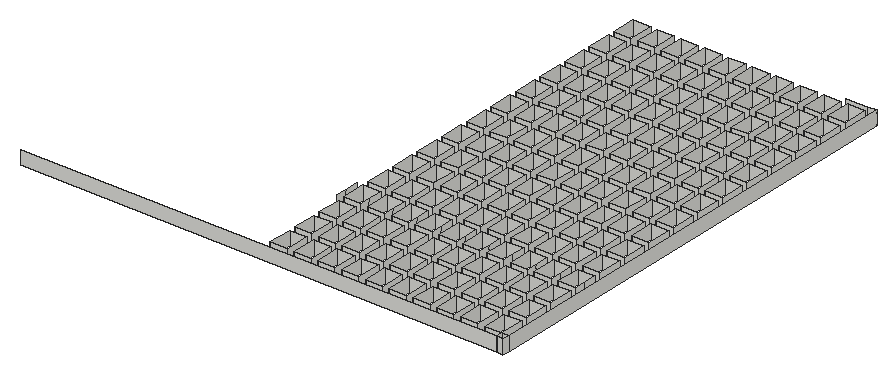
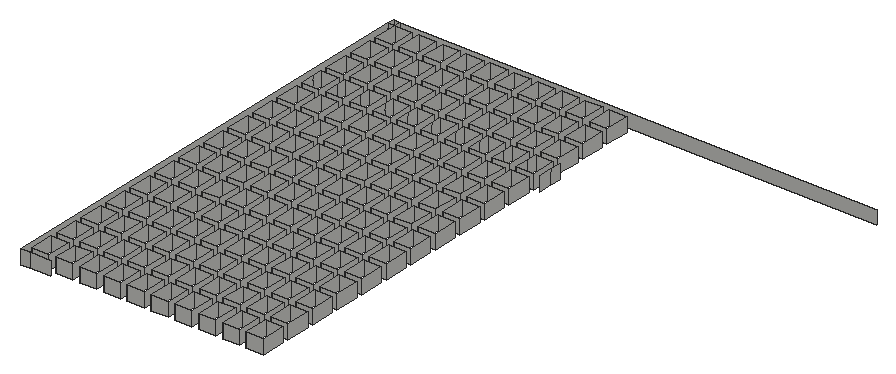
# SketchUp Ruby script. Lengths in inches.
U = 1.inch
M = Sketchup.active_model
def pt(a) = Geom::Point3d.new(a.map { |v| v * U })
def face(e, loops, mat)
  f = e.add_face(loops[0].map { |a| pt(a) })
  loops[1..].each { |l| e.add_face(l.map { |a| pt(a) }).erase! }
  f.material = f.back_material = mat if mat
  f
end
# faces: each face lists its corners as indices into pts; further lists are holes
def faces(e, pts, list, mat = nil) = list.each { |f| face(e, (f[0].is_a?(Array) ? f : [f]).map { |l| l.map { |i| pts[i] } }, mat) }
# xy, xz, yz: faces in a plane at the given z, y or x. An outline is a flat list of corners, or four numbers for a rectangle; further outlines are holes
def ring(l) = l.size == 4 ? [[l[0], l[1]], [l[2], l[1]], [l[2], l[3]], [l[0], l[3]]] : l.each_slice(2).to_a
def flat(e, list, mat, &to3) = list.each { |f| face(e, (f[0].is_a?(Array) ? f : [f]).map { |l| ring(l).map { |u, v| to3.(u, v) } }, mat) }
def xy(e, z, list, mat = nil) = flat(e, list, mat) { |x, y| [x, y, z] }
def xz(e, y, list, mat = nil) = flat(e, list, mat) { |x, z| [x, y, z] }
def yz(e, x, list, mat = nil) = flat(e, list, mat) { |y, z| [x, y, z] }
def lines(e, pts, list) = list.each { |a, b| e.add_line(pt(pts[a]), pt(pts[b])) }
# prism: a flat outline (further loops are holes) pulled along v
def prism(e, loops, v, mat = nil)
  f = face(e, loops, mat); d = Geom::Vector3d.new(v.map { |x| x * U })
  f.pushpull(f.normal.samedirection?(d) ? d.length : -d.length)
end
def box(e, o, s, mat = nil) = prism(e, [[o, [o[0] + s[0], o[1], o[2]], [o[0] + s[0], o[1] + s[1], o[2]], [o[0], o[1] + s[1], o[2]]]], [0, 0, s[2]], mat)
def at(x, y, z, deg = 0) = Geom::Transformation.translation(pt([x, y, z])) * Geom::Transformation.rotation(ORIGIN, Z_AXIS, deg.degrees)
def axes(o, x, y, z) = Geom::Transformation.new([*x, 0, *y, 0, *z, 0, *pt(o).to_a, 1])
def part(name) = M.definitions.add(name)
# library, detail: a bought-in or finely detailed component or shape, given as its bounding box
def library(name, o, s) = part(name).tap { |d| box(d.entities, o, s) }
def detail(e, o, s) = box(e.add_group.entities, o, s)
def put(e, d, t, mat = nil) = e.add_instance(d, t).tap { |i| i.material = mat if mat }
def group(e, t, mat = nil) = e.add_group.tap { |g| g.transformation = t; g.material = mat if mat }.entities
root = M.entities
xy(root,246,[[589.58,38.27,589.58,51.29,582.19,51.29,582.19,41,592.3,41,592.3,38.27]])
xz(root,38.27,[[387.37,246,589.58,252],[589.58,246,592.3,252]])
xz(root,41,[[491.2,246,498.58,252],[501.31,246,508.69,252],[511.42,246,518.8,252],[521.53,246,528.91,252],[531.64,246,539.02,252],
  [541.75,246,549.13,252],[551.86,246,559.24,252],[561.97,246,569.35,252],[572.08,246,579.47,252],[582.19,246,589.58,252],
  [589.58,246,592.3,252]])
xz(root,51.29,[[491.2,246,498.58,252],[501.31,246,508.69,252],[511.42,246,518.8,252],[521.53,246,528.91,252],[531.64,246,539.02,252],
  [541.75,246,549.13,252],[551.86,246,559.24,252],[561.97,246,569.35,252],[572.08,246,579.47,252],[582.19,246,589.58,252]])
xz(root,54.01,[[491.2,246,498.58,252],[501.31,246,508.69,252],[511.42,246,518.8,252],[521.53,246,528.91,252],[531.64,246,539.02,252],
  [541.75,246,549.13,252],[551.86,246,559.24,252],[561.97,246,569.35,252],[572.08,246,579.47,252],[582.19,246,589.58,252]])
xz(root,64.3,[[491.2,246,498.58,252],[501.31,246,508.69,252],[511.42,246,518.8,252],[521.53,246,528.91,252],[531.64,246,539.02,252],
  [541.75,246,549.13,252],[551.86,246,559.24,252],[561.97,246,569.35,252],[572.08,246,579.47,252],[582.19,246,589.58,252]])
xz(root,67.02,[[491.2,246,498.58,252],[501.31,246,508.69,252],[511.42,246,518.8,252],[521.53,246,528.91,252],[531.64,246,539.02,252],
  [541.75,246,549.13,252],[551.86,246,559.24,252],[561.97,246,569.35,252],[572.08,246,579.47,252],[582.19,246,589.58,252]])
xz(root,77.31,[[491.2,246,498.58,252],[501.31,246,508.69,252],[511.42,246,518.8,252],[521.53,246,528.91,252],[531.64,246,539.02,252],
  [541.75,246,549.13,252],[551.86,246,559.24,252],[561.97,246,569.35,252],[572.08,246,579.47,252],[582.19,246,589.58,252]])
xz(root,80.03,[[491.2,246,498.58,252],[501.31,246,508.69,252],[511.42,246,518.8,252],[521.53,246,528.91,252],[531.64,246,539.02,252],
  [541.75,246,549.13,252],[551.86,246,559.24,252],[561.97,246,569.35,252],[572.08,246,579.47,252],[582.19,246,589.58,252]])
xz(root,90.32,[[491.2,246,498.58,252],[501.31,246,508.69,252],[511.42,246,518.8,252],[521.53,246,528.91,252],[531.64,246,539.02,252],
  [541.75,246,549.13,252],[551.86,246,559.24,252],[561.97,246,569.35,252],[572.08,246,579.47,252],[582.19,246,589.58,252]])
xz(root,93.05,[[491.2,246,498.58,252],[501.31,246,508.69,252],[511.42,246,518.8,252],[521.53,246,528.91,252],[531.64,246,539.02,252],
  [541.75,246,549.13,252],[551.86,246,559.24,252],[561.97,246,569.35,252],[572.08,246,579.47,252],[582.19,246,589.58,252]])
xz(root,103.33,[[491.2,246,498.58,252],[501.31,246,508.69,252],[511.42,246,518.8,252],[521.53,246,528.91,252],[531.64,246,539.02,252],
  [541.75,246,549.13,252],[551.86,246,559.24,252],[561.97,246,569.35,252],[572.08,246,579.47,252],[582.19,246,589.58,252]])
xz(root,106.06,[[491.2,246,498.58,252],[501.31,246,508.69,252],[511.42,246,518.8,252],[521.53,246,528.91,252],[531.64,246,539.02,252],
  [541.75,246,549.13,252],[551.86,246,559.24,252],[561.97,246,569.35,252],[572.08,246,579.47,252],[582.19,246,589.58,252]])
xz(root,116.34,[[491.2,246,498.58,252],[501.31,246,508.69,252],[511.42,246,518.8,252],[521.53,246,528.91,252],[531.64,246,539.02,252],
  [541.75,246,549.13,252],[551.86,246,559.24,252],[561.97,246,569.35,252],[572.08,246,579.47,252],[582.19,246,589.58,252]])
xz(root,119.07,[[491.2,246,498.58,252],[501.31,246,508.69,252],[511.42,246,518.8,252],[521.53,246,528.91,252],[531.64,246,539.02,252],
  [541.75,246,549.13,252],[551.86,246,559.24,252],[561.97,246,569.35,252],[572.08,246,579.47,252],[582.19,246,589.58,252]])
xz(root,129.36,[[491.2,246,498.58,252],[501.31,246,508.69,252],[511.42,246,518.8,252],[521.53,246,528.91,252],[531.64,246,539.02,252],
  [541.75,246,549.13,252],[551.86,246,559.24,252],[561.97,246,569.35,252],[572.08,246,579.47,252],[582.19,246,589.58,252]])
xz(root,132.08,[[491.2,246,498.58,252],[501.31,246,508.69,252],[511.42,246,518.8,252],[521.53,246,528.91,252],[531.64,246,539.02,252],
  [541.75,246,549.13,252],[551.86,246,559.24,252],[561.97,246,569.35,252],[572.08,246,579.47,252],[582.19,246,589.58,252]])
xz(root,142.37,[[491.2,246,498.58,252],[501.31,246,508.69,252],[511.42,246,518.8,252],[521.53,246,528.91,252],[531.64,246,539.02,252],
  [541.75,246,549.13,252],[551.86,246,559.24,252],[561.97,246,569.35,252],[572.08,246,579.47,252],[582.19,246,589.58,252]])
xz(root,145.09,[[491.2,246,498.58,252],[501.31,246,508.69,252],[511.42,246,518.8,252],[521.53,246,528.91,252],[531.64,246,539.02,252],
  [541.75,246,549.13,252],[551.86,246,559.24,252],[561.97,246,569.35,252],[572.08,246,579.47,252],[582.19,246,589.58,252]])
xz(root,155.38,[[491.2,246,498.58,252],[501.31,246,508.69,252],[511.42,246,518.8,252],[521.53,246,528.91,252],[531.64,246,539.02,252],
  [541.75,246,549.13,252],[551.86,246,559.24,252],[561.97,246,569.35,252],[572.08,246,579.47,252],[582.19,246,589.58,252]])
xz(root,158.1,[[491.2,246,498.58,252],[501.31,246,508.69,252],[511.42,246,518.8,252],[521.53,246,528.91,252],[531.64,246,539.02,252],
  [541.75,246,549.13,252],[551.86,246,559.24,252],[561.97,246,569.35,252],[572.08,246,579.47,252],[582.19,246,589.58,252]])
xz(root,168.39,[[491.2,246,498.58,252],[501.31,246,508.69,252],[511.42,246,518.8,252],[521.53,246,528.91,252],[531.64,246,539.02,252],
  [541.75,246,549.13,252],[551.86,246,559.24,252],[561.97,246,569.35,252],[572.08,246,579.47,252],[582.19,246,589.58,252]])
xz(root,171.12,[[491.2,246,498.58,252],[501.31,246,508.69,252],[511.42,246,518.8,252],[521.53,246,528.91,252],[531.64,246,539.02,252],
  [541.75,246,549.13,252],[551.86,246,559.24,252],[561.97,246,569.35,252],[572.08,246,579.47,252],[582.19,246,589.58,252]])
xz(root,181.4,[[491.2,246,498.58,252],[501.31,246,508.69,252],[511.42,246,518.8,252],[521.53,246,528.91,252],[531.64,246,539.02,252],
  [541.75,246,549.13,252],[551.86,246,559.24,252],[561.97,246,569.35,252],[572.08,246,579.47,252],[582.19,246,589.58,252]])
xz(root,184.13,[[491.2,246,498.58,252],[501.31,246,508.69,252],[511.42,246,518.8,252],[521.53,246,528.91,252],[531.64,246,539.02,252],
  [541.75,246,549.13,252],[551.86,246,559.24,252],[561.97,246,569.35,252],[572.08,246,579.47,252],[582.19,246,589.58,252]])
xz(root,194.41,[[491.2,246,498.58,252],[501.31,246,508.69,252],[511.42,246,518.8,252],[521.53,246,528.91,252],[531.64,246,539.02,252],
  [541.75,246,549.13,252],[551.86,246,559.24,252],[561.97,246,569.35,252],[572.08,246,579.47,252],[582.19,246,589.58,252]])
xz(root,197.14,[[491.2,246,498.58,252],[501.31,246,508.69,252],[511.42,246,518.8,252],[521.53,246,528.91,252],[531.64,246,539.02,252],
  [541.75,246,549.13,252],[551.86,246,559.24,252],[561.97,246,569.35,252],[572.08,246,579.47,252],[582.19,246,589.58,252]])
xz(root,207.43,[[491.2,246,498.58,252],[501.31,246,508.69,252],[511.42,246,518.8,252],[521.53,246,528.91,252],[531.64,246,539.02,252],
  [541.75,246,549.13,252],[551.86,246,559.24,252],[561.97,246,569.35,252],[572.08,246,579.47,252],[582.19,246,589.58,252]])
xz(root,210.15,[[491.2,246,498.58,252],[501.31,246,508.69,252],[511.42,246,518.8,252],[521.53,246,528.91,252],[531.64,246,539.02,252],
  [541.75,246,549.13,252],[551.86,246,559.24,252],[561.97,246,569.35,252],[572.08,246,579.47,252],[582.19,246,589.58,252]])
xz(root,220.4375,[[491.2,246,498.58,252],[501.31,246,508.69,252],[511.42,246,518.8,252],[521.53,246,528.91,252],[531.64,246,539.02,252],
  [541.75,246,549.13,252],[551.86,246,559.24,252],[561.97,246,569.35,252],[572.08,246,579.47,252],[582.19,246,589.58,252]])
xz(root,223.16,[[491.2,246,498.58,252],[501.31,246,508.69,252],[511.42,246,518.8,252],[521.53,246,528.91,252],[531.64,246,539.02,252],
  [541.75,246,549.13,252],[551.86,246,559.24,252],[561.97,246,569.35,252],[572.08,246,579.47,252],[582.19,246,589.58,252]])
xz(root,233.45,[[491.2,246,498.58,252],[501.31,246,508.69,252],[511.42,246,518.8,252],[521.53,246,528.91,252],[531.64,246,539.02,252],
  [541.75,246,549.13,252],[551.86,246,559.24,252],[561.97,246,569.35,252],[572.08,246,579.47,252],[582.19,246,589.58,252]])
xz(root,236.18,[[579.37,246,588.37,252],[588.37,246,592.3,252]])
yz(root,488.47,[[80.03,246,84.36,252],[84.36,246,90.32,252]])
yz(root,491.2,[[41,246,51.29,252],[54.01,246,64.3,252],[67.02,246,77.31,252],[80.03,246,90.32,252],[93.05,246,103.33,252],
  [106.06,246,116.34,252],[119.07,246,129.36,252],[132.08,246,142.37,252],[145.09,246,155.38,252],[158.1,246,168.39,252],
  [171.12,246,181.4,252],[184.13,246,194.41,252],[197.14,246,207.43,252],[210.15,246,220.4375,252],[223.16,246,233.45,252]])
yz(root,498.58,[[41,246,51.29,252],[54.01,246,64.3,252],[67.02,246,77.31,252],[80.03,246,84.36,252],[84.36,246,90.32,252],
  [93.05,246,103.33,252],[106.06,246,116.34,252],[119.07,246,129.36,252],[132.08,246,142.37,252],[145.09,246,155.38,252],
  [158.1,246,168.39,252],[171.12,246,181.4,252],[184.13,246,194.41,252],[197.14,246,207.43,252],[210.15,246,220.4375,252],
  [223.16,246,233.45,252]])
yz(root,501.31,[[41,246,51.29,252],[54.01,246,64.3,252],[67.02,246,77.31,252],[80.03,246,90.32,252],[93.05,246,103.33,252],
  [106.06,246,116.34,252],[119.07,246,129.36,252],[132.08,246,142.37,252],[145.09,246,155.38,252],[158.1,246,168.39,252],
  [171.12,246,181.4,252],[184.13,246,194.41,252],[197.14,246,207.43,252],[210.15,246,220.4375,252],[223.16,246,233.45,252]])
yz(root,508.69,[[41,246,51.29,252],[54.01,246,64.3,252],[67.02,246,77.31,252],[80.03,246,84.36,252],[84.36,246,90.32,252],
  [93.05,246,103.33,252],[106.06,246,116.34,252],[119.07,246,129.36,252],[132.08,246,142.37,252],[145.09,246,155.38,252],
  [158.1,246,168.39,252],[171.12,246,181.4,252],[184.13,246,194.41,252],[197.14,246,207.43,252],[210.15,246,220.4375,252],
  [223.16,246,233.45,252]])
yz(root,511.42,[[41,246,51.29,252],[54.01,246,64.3,252],[67.02,246,77.31,252],[80.03,246,90.32,252],[93.05,246,103.33,252],
  [106.06,246,116.34,252],[119.07,246,129.36,252],[132.08,246,142.37,252],[145.09,246,155.38,252],[158.1,246,168.39,252],
  [171.12,246,181.4,252],[184.13,246,194.41,252],[197.14,246,207.43,252],[210.15,246,220.4375,252],[223.16,246,233.45,252]])
yz(root,518.8,[[41,246,51.29,252],[54.01,246,64.3,252],[67.02,246,77.31,252],[80.03,246,84.36,252],[84.36,246,90.32,252],
  [93.05,246,103.33,252],[106.06,246,116.34,252],[119.07,246,129.36,252],[132.08,246,142.37,252],[145.09,246,155.38,252],
  [158.1,246,168.39,252],[171.12,246,181.4,252],[184.13,246,194.41,252],[197.14,246,207.43,252],[210.15,246,220.4375,252],
  [223.16,246,233.45,252]])
yz(root,521.53,[[41,246,51.29,252],[54.01,246,64.3,252],[67.02,246,77.31,252],[80.03,246,90.32,252],[93.05,246,103.33,252],
  [106.06,246,116.34,252],[119.07,246,129.36,252],[132.08,246,142.37,252],[145.09,246,155.38,252],[158.1,246,168.39,252],
  [171.12,246,181.4,252],[184.13,246,194.41,252],[197.14,246,207.43,252],[210.15,246,220.4375,252],[223.16,246,233.45,252]])
yz(root,528.91,[[41,246,51.29,252],[54.01,246,64.3,252],[67.02,246,77.31,252],[80.03,246,84.36,252],[84.36,246,90.32,252],
  [93.05,246,103.33,252],[106.06,246,116.34,252],[119.07,246,129.36,252],[132.08,246,142.37,252],[145.09,246,155.38,252],
  [158.1,246,168.39,252],[171.12,246,181.4,252],[184.13,246,194.41,252],[197.14,246,207.43,252],[210.15,246,220.4375,252],
  [223.16,246,233.45,252]])
yz(root,531.64,[[41,246,51.29,252],[54.01,246,64.3,252],[67.02,246,77.31,252],[80.03,246,90.32,252],[93.05,246,103.33,252],
  [106.06,246,116.34,252],[119.07,246,129.36,252],[132.08,246,142.37,252],[145.09,246,155.38,252],[158.1,246,168.39,252],
  [171.12,246,181.4,252],[184.13,246,194.41,252],[197.14,246,207.43,252],[210.15,246,220.4375,252],[223.16,246,233.45,252]])
yz(root,539.02,[[41,246,51.29,252],[54.01,246,64.3,252],[67.02,246,77.31,252],[80.03,246,84.36,252],[84.36,246,90.32,252],
  [93.05,246,103.33,252],[106.06,246,116.34,252],[119.07,246,129.36,252],[132.08,246,142.37,252],[145.09,246,155.38,252],
  [158.1,246,168.39,252],[171.12,246,181.4,252],[184.13,246,194.41,252],[197.14,246,207.43,252],[210.15,246,220.4375,252],
  [223.16,246,233.45,252]])
yz(root,541.75,[[41,246,51.29,252],[54.01,246,64.3,252],[67.02,246,77.31,252],[80.03,246,90.32,252],[93.05,246,103.33,252],
  [106.06,246,116.34,252],[119.07,246,129.36,252],[132.08,246,142.37,252],[145.09,246,155.38,252],[158.1,246,168.39,252],
  [171.12,246,181.4,252],[184.13,246,194.41,252],[197.14,246,207.43,252],[210.15,246,220.4375,252],[223.16,246,233.45,252]])
yz(root,549.13,[[41,246,51.29,252],[54.01,246,64.3,252],[67.02,246,77.31,252],[80.03,246,84.36,252],[84.36,246,90.32,252],
  [93.05,246,103.33,252],[106.06,246,116.34,252],[119.07,246,129.36,252],[132.08,246,142.37,252],[145.09,246,155.38,252],
  [158.1,246,168.39,252],[171.12,246,181.4,252],[184.13,246,194.41,252],[197.14,246,207.43,252],[210.15,246,220.4375,252],
  [223.16,246,233.45,252]])
yz(root,551.86,[[41,246,51.29,252],[54.01,246,64.3,252],[67.02,246,77.31,252],[80.03,246,90.32,252],[93.05,246,103.33,252],
  [106.06,246,116.34,252],[119.07,246,129.36,252],[132.08,246,142.37,252],[145.09,246,155.38,252],[158.1,246,168.39,252],
  [171.12,246,181.4,252],[184.13,246,194.41,252],[197.14,246,207.43,252],[210.15,246,220.4375,252],[223.16,246,233.45,252]])
yz(root,559.24,[[41,246,51.29,252],[54.01,246,64.3,252],[67.02,246,77.31,252],[80.03,246,84.36,252],[84.36,246,90.32,252],
  [93.05,246,103.33,252],[106.06,246,116.34,252],[119.07,246,129.36,252],[132.08,246,142.37,252],[145.09,246,155.38,252],
  [158.1,246,168.39,252],[171.12,246,181.4,252],[184.13,246,194.41,252],[197.14,246,207.43,252],[210.15,246,220.4375,252],
  [223.16,246,233.45,252]])
yz(root,561.97,[[41,246,51.29,252],[54.01,246,64.3,252],[67.02,246,77.31,252],[80.03,246,90.32,252],[93.05,246,103.33,252],
  [106.06,246,116.34,252],[119.07,246,129.36,252],[132.08,246,142.37,252],[145.09,246,155.38,252],[158.1,246,168.39,252],
  [171.12,246,181.4,252],[184.13,246,194.41,252],[197.14,246,207.43,252],[210.15,246,220.4375,252],[223.16,246,233.45,252]])
yz(root,569.35,[[41,246,51.29,252],[54.01,246,64.3,252],[67.02,246,77.31,252],[80.03,246,84.36,252],[84.36,246,90.32,252],
  [93.05,246,103.33,252],[106.06,246,116.34,252],[119.07,246,129.36,252],[132.08,246,142.37,252],[145.09,246,155.38,252],
  [158.1,246,168.39,252],[171.12,246,181.4,252],[184.13,246,194.41,252],[197.14,246,207.43,252],[210.15,246,220.4375,252],
  [223.16,246,233.45,252]])
yz(root,572.08,[[41,246,51.29,252],[54.01,246,64.3,252],[67.02,246,77.31,252],[80.03,246,90.32,252],[93.05,246,103.33,252],
  [106.06,246,116.34,252],[119.07,246,129.36,252],[132.08,246,142.37,252],[145.09,246,155.38,252],[158.1,246,168.39,252],
  [171.12,246,181.4,252],[184.13,246,194.41,252],[197.14,246,207.43,252],[210.15,246,220.4375,252],[223.16,246,233.45,252]])
yz(root,579.47,[[41,246,51.29,252],[54.01,246,64.3,252],[67.02,246,77.31,252],[80.03,246,84.36,252],[84.36,246,90.32,252],
  [93.05,246,103.33,252],[106.06,246,116.34,252],[119.07,246,129.36,252],[132.08,246,142.37,252],[145.09,246,155.38,252],
  [158.1,246,168.39,252],[171.12,246,181.4,252],[184.13,246,194.41,252],[197.14,246,207.43,252],[210.15,246,220.4375,252],
  [223.16,246,233.45,252]])
yz(root,582.19,[[41,246,51.29,252],[54.01,246,64.3,252],[67.02,246,77.31,252],[80.03,246,90.32,252],[93.05,246,103.33,252],
  [106.06,246,116.34,252],[119.07,246,129.36,252],[132.08,246,142.37,252],[145.09,246,155.38,252],[158.1,246,168.39,252],
  [171.12,246,181.4,252],[184.13,246,194.41,252],[197.14,246,207.43,252],[210.15,246,220.4375,252],[223.16,246,233.45,252]])
yz(root,589.58,[[38.27,246,41,252],[41,246,51.29,252],[54.01,246,64.3,252],[67.02,246,77.31,252],[80.03,246,84.36,252],
  [84.36,246,90.32,252],[93.05,246,103.33,252],[106.06,246,116.34,252],[119.07,246,129.36,252],[132.08,246,142.37,252],
  [145.09,246,155.38,252],[158.1,246,168.39,252],[171.12,246,181.4,252],[184.13,246,194.41,252],[197.14,246,207.43,252],
  [210.15,246,220.4375,252],[223.16,246,233.45,252]])
yz(root,592.3,[[38.27,246,41,252],[41,246,236.18,252]])
